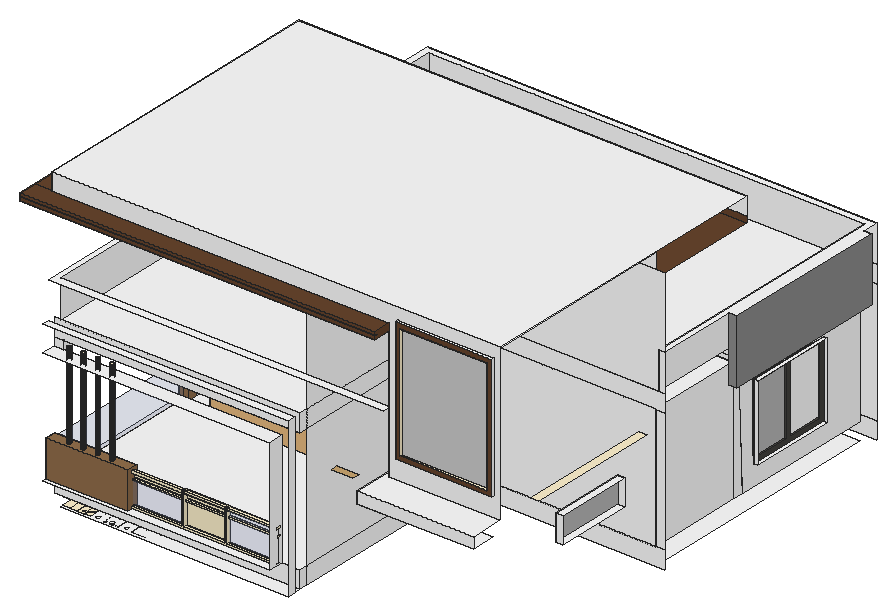
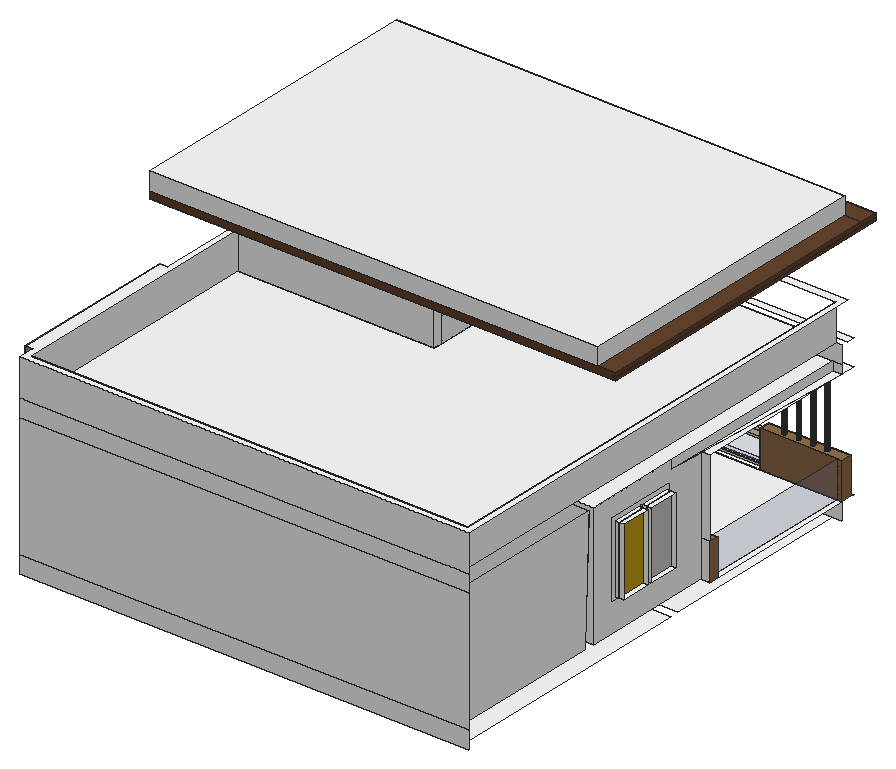
# SketchUp Ruby script. Lengths in inches.
U = 1.inch
M = Sketchup.active_model
def pt(a) = Geom::Point3d.new(a.map { |v| v * U })
def face(e, loops, mat)
  f = e.add_face(loops[0].map { |a| pt(a) })
  loops[1..].each { |l| e.add_face(l.map { |a| pt(a) }).erase! }
  f.material = f.back_material = mat if mat
  f
end
# faces: each face lists its corners as indices into pts; further lists are holes
def faces(e, pts, list, mat = nil) = list.each { |f| face(e, (f[0].is_a?(Array) ? f : [f]).map { |l| l.map { |i| pts[i] } }, mat) }
# xy, xz, yz: faces in a plane at the given z, y or x. An outline is a flat list of corners, or four numbers for a rectangle; further outlines are holes
def ring(l) = l.size == 4 ? [[l[0], l[1]], [l[2], l[1]], [l[2], l[3]], [l[0], l[3]]] : l.each_slice(2).to_a
def flat(e, list, mat, &to3) = list.each { |f| face(e, (f[0].is_a?(Array) ? f : [f]).map { |l| ring(l).map { |u, v| to3.(u, v) } }, mat) }
def xy(e, z, list, mat = nil) = flat(e, list, mat) { |x, y| [x, y, z] }
def xz(e, y, list, mat = nil) = flat(e, list, mat) { |x, z| [x, y, z] }
def yz(e, x, list, mat = nil) = flat(e, list, mat) { |y, z| [x, y, z] }
def lines(e, pts, list) = list.each { |a, b| e.add_line(pt(pts[a]), pt(pts[b])) }
# prism: a flat outline (further loops are holes) pulled along v
def prism(e, loops, v, mat = nil)
  f = face(e, loops, mat); d = Geom::Vector3d.new(v.map { |x| x * U })
  f.pushpull(f.normal.samedirection?(d) ? d.length : -d.length)
end
def box(e, o, s, mat = nil) = prism(e, [[o, [o[0] + s[0], o[1], o[2]], [o[0] + s[0], o[1] + s[1], o[2]], [o[0], o[1] + s[1], o[2]]]], [0, 0, s[2]], mat)
def at(x, y, z, deg = 0) = Geom::Transformation.translation(pt([x, y, z])) * Geom::Transformation.rotation(ORIGIN, Z_AXIS, deg.degrees)
def axes(o, x, y, z) = Geom::Transformation.new([*x, 0, *y, 0, *z, 0, *pt(o).to_a, 1])
def part(name) = M.definitions.add(name)
# library, detail: a bought-in or finely detailed component or shape, given as its bounding box
def library(name, o, s) = part(name).tap { |d| box(d.entities, o, s) }
def detail(e, o, s) = box(e.add_group.entities, o, s)
def put(e, d, t, mat = nil) = e.add_instance(d, t).tap { |i| i.material = mat if mat }
def group(e, t, mat = nil) = e.add_group.tap { |g| g.transformation = t; g.material = mat if mat }.entities
root = M.entities
M.materials.add("D01_Frost_White").color = [255, 242, 206]
M.materials.add("Glass_Mirror_01").color = [185, 185, 185]
M.materials.add("Glass_Sky Reflection_01").color = [126, 138, 183]
M.materials["Glass_Sky Reflection_01"].alpha = 0.25
M.materials.add("M00_Soft_Cloud").color = [255, 255, 255]
M.materials.add("M04_Stone_Frost").color = [142, 142, 142]
M.materials.add("Metal_06_1K").color = [238, 236, 231]
M.materials.add("Metal_Perforated_03_1K").color = [205, 205, 205]
M.materials.add("Metal_Perforated_08_1K").color = [201, 163, 22]
M.materials.add("Plywood_08_1K").color = [202, 166, 113]
M.materials.add("Wood_Floor_01_1K").color = [146, 111, 76]
M.materials.add("Wood_Planks_01_1K").color = [69, 67, 63]
M.materials.add("Wood_Veneer_15_1K1").color = [103, 69, 45]
c1 = library("michel-club1 (1)",[-34.67,-0.85,-0.13],[126.28,91.17,33.41])
xy(root,257.001,[[209.9258,109.0676,209.9294,119.6039],[209.933,109.0676,216.6168,119.6039],[216.6168,109.0676,223.3077,119.6039]],"D01_Frost_White")
xy(root,257.004,[[183.1639,109.0676,189.8512,119.6039],[189.8548,109.0676,196.5422,119.6039],[196.5529,109.0676,196.5547,119.6039]],"D01_Frost_White")
xy(root,257.0071,[[183.1621,109.0676,183.1657,119.6039],[196.5511,109.0676,203.242,119.6039],[203.242,109.0676,209.933,119.6039]],"D01_Frost_White")
xy(root,257.0132,[[169.7874,109.0676,176.4783,119.6039],[176.4783,109.0676,183.1692,119.6039]],"D01_Frost_White")
xy(root,257.0192,[[143.0236,109.0676,149.7146,119.6039],[149.7146,109.0676,156.4019,119.6039],[156.4055,109.0676,163.0929,119.6039],[163.0929,109.0676,169.7838,119.6039]],"D01_Frost_White")
xy(root,257.0192,[[[143.4397,105.8195,366,120],[190.0131,108.9163,189.5258,108.9804,189.0716,109.1685,188.6816,109.4678,188.3824,109.8578,188.1943,110.3119,188.1301,110.7993,188.1943,111.2867,188.3824,111.7408,188.6816,112.1308,189.0716,112.43,189.5258,112.6182,190.0131,112.6823,190.5005,112.6182,190.9547,112.43,191.3446,112.1308,191.6439,111.7408,191.832,111.2867,191.8962,110.7993,191.832,110.3119,191.6439,109.8578,191.3446,109.4678,190.9547,109.1685,190.5005,108.9804],[203.9218,108.9163,203.4345,108.9804,202.9803,109.1685,202.5903,109.4678,202.2911,109.8578,202.103,110.3119,202.0388,110.7993,202.103,111.2867,202.2911,111.7408,202.5903,112.1308,202.9803,112.43,203.4345,112.6182,203.9218,112.6823,204.4092,112.6182,204.8634,112.43,205.2534,112.1308,205.5526,111.7408,205.7407,111.2867,205.8049,110.7993,205.7407,110.3119,205.5526,109.8578,205.2534,109.4678,204.8634,109.1685,204.4092,108.9804],[162.1957,108.9163,161.7084,108.9804,161.2542,109.1685,160.8642,109.4678,160.565,109.8578,160.3769,110.3119,160.3127,110.7993,160.3769,111.2867,160.565,111.7408,160.8642,112.1308,161.2542,112.43,161.7084,112.6182,162.1957,112.6823,162.6831,112.6182,163.1373,112.43,163.5272,112.1308,163.8265,111.7408,164.0146,111.2867,164.0788,110.7993,164.0146,110.3119,163.8265,109.8578,163.5272,109.4678,163.1373,109.1685,162.6831,108.9804],[176.1044,108.9163,175.6171,108.9804,175.1629,109.1685,174.7729,109.4678,174.4737,109.8578,174.2856,110.3119,174.2214,110.7993,174.2856,111.2867,174.4737,111.7408,174.7729,112.1308,175.1629,112.43,175.6171,112.6182,176.1044,112.6823,176.5918,112.6182,177.046,112.43,177.4359,112.1308,177.7352,111.7408,177.9233,111.2867,177.9875,110.7993,177.9233,110.3119,177.7352,109.8578,177.4359,109.4678,177.046,109.1685,176.5918,108.9804]],[162.1957,108.9163,162.6831,108.9804,163.1373,109.1685,163.5272,109.4678,163.8265,109.8578,164.0146,110.3119,164.0788,110.7993,164.0146,111.2867,163.8265,111.7408,163.5272,112.1308,163.1373,112.43,162.6831,112.6182,162.1957,112.6823,161.7084,112.6182,161.2542,112.43,160.8642,112.1308,160.565,111.7408,160.3769,111.2867,160.3127,110.7993,160.3769,110.3119,160.565,109.8578,160.8642,109.4678,161.2542,109.1685,161.7084,108.9804],[176.1044,108.9163,176.5918,108.9804,177.046,109.1685,177.4359,109.4678,177.7352,109.8578,177.9233,110.3119,177.9875,110.7993,177.9233,111.2867,177.7352,111.7408,177.4359,112.1308,177.046,112.43,176.5918,112.6182,176.1044,112.6823,175.6171,112.6182,175.1629,112.43,174.7729,112.1308,174.4737,111.7408,174.2856,111.2867,174.2214,110.7993,174.2856,110.3119,174.4737,109.8578,174.7729,109.4678,175.1629,109.1685,175.6171,108.9804],[190.0131,108.9163,190.5005,108.9804,190.9547,109.1685,191.3446,109.4678,191.6439,109.8578,191.832,110.3119,191.8962,110.7993,191.832,111.2867,191.6439,111.7408,191.3446,112.1308,190.9547,112.43,190.5005,112.6182,190.0131,112.6823,189.5258,112.6182,189.0716,112.43,188.6816,112.1308,188.3824,111.7408,188.1943,111.2867,188.1301,110.7993,188.1943,110.3119,188.3824,109.8578,188.6816,109.4678,189.0716,109.1685,189.5258,108.9804],[203.9218,108.9163,204.4092,108.9804,204.8634,109.1685,205.2534,109.4678,205.5526,109.8578,205.7407,110.3119,205.8049,110.7993,205.7407,111.2867,205.5526,111.7408,205.2534,112.1308,204.8634,112.43,204.4092,112.6182,203.9218,112.6823,203.4345,112.6182,202.9803,112.43,202.5903,112.1308,202.2911,111.7408,202.103,111.2867,202.0388,110.7993,202.103,110.3119,202.2911,109.8578,202.5903,109.4678,202.9803,109.1685,203.4345,108.9804],
  [135,120,366,309],[135,318,555,567]],"M00_Soft_Cloud")
xy(root,274.0384,[[126,105.8195,348,105.8195,348,120,205.8751,120,205.8751,109.5496,126,109.5496],[126,109.5496,205.8751,120],[126,120,130.5,272.2237],[130.5,120,366,120,366,412.2579,135,412.2579,135,272.2237,130.5,272.2237],[126,272.2237,135,281.2237],
  [378.0564,318,555,412.2579]],"M00_Soft_Cloud")
xy(root,274.5723,[[205.8751,113.3173,348.7066,116.9059]],"D01_Frost_White")
xy(root,276.5176,[[205.8751,113.3173,255.4424,115.614],[257.6603,113.3173,297.4834,116.9059],[299.7013,113.3173,348.7066,115.1116],[299.7013,115.1116,348.7066,116.9059],[205.8751,115.614,255.4424,116.9059]],"D01_Frost_White")
xy(root,282.3496,[[366,337.9558,372.0282,371.4203],[372.0282,337.9558,378.0564,371.4203]],"M00_Soft_Cloud")
xy(root,298.6563,[[205.8751,114.3221,348.7066,116.9059]],"D01_Frost_White")
xy(root,298.8738,[[560.4663,430.9412,564,515.7903]],"M00_Soft_Cloud")
xy(root,300.1736,[[205.8751,114.3221,348.7066,116.9059]],"D01_Frost_White")
xy(root,302.8738,[[555,434.9412,557.7332,471.3657],[555,475.3657,557.7332,511.7903]],"M00_Soft_Cloud")
xy(root,302.8738,[[557.7332,434.9412,560.4663,471.3657],[557.7332,475.3657,560.4663,511.7903]],"Wood_Planks_01_1K")
xy(root,304.975,[[126,323.2546,130.5,353.0052],[130.5,323.2546,135,353.0052],[126,357.0052,130.5,386.7557],[130.5,357.0052,135,386.7557]],"M00_Soft_Cloud")
xy(root,305.9572,[[205.8751,113.3173,348.7066,116.9059]],"D01_Frost_White")
xy(root,307.9026,[[205.8751,113.3173,255.4424,116.9059],[255.4424,113.3173,257.6603,116.9059],[257.6603,113.3173,297.4834,116.9059],[297.4834,113.3173,299.7013,116.9059],[299.7013,113.3173,348.7066,116.9059]],"D01_Frost_White")
xy(root,310.0384,[[[126,109.5496,205.8751,120],[144.756,112.6463,144.2686,112.7104,143.8145,112.8986,143.4245,113.1978,143.1252,113.5878,142.9371,114.0419,142.873,114.5293,142.9371,115.0167,143.1252,115.4708,143.4245,115.8608,143.8145,116.1601,144.2686,116.3482,144.756,116.4123,145.2434,116.3482,145.6975,116.1601,146.0875,115.8608,146.3868,115.4708,146.5749,115.0167,146.639,114.5293,146.5749,114.0419,146.3868,113.5878,146.0875,113.1978,145.6975,112.8986,145.2434,112.7104],[158.6647,112.6463,158.1773,112.7104,157.7232,112.8986,157.3332,113.1978,157.034,113.5878,156.8458,114.0419,156.7817,114.5293,156.8458,115.0167,157.034,115.4708,157.3332,115.8608,157.7232,116.1601,158.1773,116.3482,158.6647,116.4123,159.1521,116.3482,159.6062,116.1601,159.9962,115.8608,160.2955,115.4708,160.4836,115.0167,160.5477,114.5293,160.4836,114.0419,160.2955,113.5878,159.9962,113.1978,159.6062,112.8986,159.1521,112.7104],[172.5734,112.6463,172.086,112.7104,171.6319,112.8986,171.2419,113.1978,170.9427,113.5878,170.7545,114.0419,170.6904,114.5293,170.7545,115.0167,170.9427,115.4708,171.2419,115.8608,171.6319,116.1601,172.086,116.3482,172.5734,116.4123,173.0608,116.3482,173.5149,116.1601,173.9049,115.8608,174.2042,115.4708,174.3923,115.0167,174.4564,114.5293,174.3923,114.0419,174.2042,113.5878,173.9049,113.1978,173.5149,112.8986,173.0608,112.7104],[186.4821,112.6463,185.9947,112.7104,185.5406,112.8986,185.1506,113.1978,184.8514,113.5878,184.6632,114.0419,184.5991,114.5293,184.6632,115.0167,184.8514,115.4708,185.1506,115.8608,185.5406,116.1601,185.9947,116.3482,186.4821,116.4123,186.9695,116.3482,187.4236,116.1601,187.8136,115.8608,188.1129,115.4708,188.301,115.0167,188.3651,114.5293,188.301,114.0419,188.1129,113.5878,187.8136,113.1978,187.4236,112.8986,186.9695,112.7104]],[126,272.2237,135,281.2237]],"Wood_Floor_01_1K")
xy(root,339.7221,[[564,184.6361,571,259.8187]],"M00_Soft_Cloud")
xy(root,364.3605,[[463.5996,116.0568,528.8247,122.5284],[463.5996,122.5284,528.8247,129]],"M00_Soft_Cloud")
xy(root,365.0444,[[564,184.6361,571,259.8187]],"M00_Soft_Cloud")
xy(root,368.9179,[[555,434.9412,557.7332,471.3657],[555,475.3657,557.7332,511.7903]],"M00_Soft_Cloud")
xy(root,368.9179,[[557.7332,434.9412,560.4663,471.3657],[557.7332,475.3657,560.4663,511.7903]],"Wood_Planks_01_1K")
xy(root,371.0202,[[366,337.9558,372.0282,371.4203],[372.0282,337.9558,378.0564,371.4203]],"M00_Soft_Cloud")
xy(root,371.1879,[[126,323.2546,130.5,353.0052],[130.5,323.2546,135,353.0052],[126,357.0052,130.5,386.7557],[130.5,357.0052,135,386.7557]],"M00_Soft_Cloud")
xy(root,372.3605,[[455.5996,116.0568,536.8247,128.0311]],"M00_Soft_Cloud")
xy(root,372.9179,[[560.4663,430.9412,564,515.7903]],"M00_Soft_Cloud")
xy(root,377.4389,[[450.4407,84.0124,450.4407,128.0311,546,128.0311,546,108.0124,564,108.0124,564,84.0124]],"M00_Soft_Cloud")
xy(root,377.6765,[[402.037,112.9098,423.1418,120]],"Plywood_08_1K")
xy(root,384.3022,[[564,396.1656,571.6233,560.6941]],"M04_Stone_Frost")
xy(root,385.4776,[[126,105.8195,348,120]],"M00_Soft_Cloud")
xy(root,388.7049,[[450.4407,84.0124,564,84.0124,564,116.3941,455.5996,116.3941,455.5996,128.0311,450.4407,128.0311]],"M00_Soft_Cloud")
xy(root,390.9895,[[564,154.6118,571,286.5421]],"D01_Frost_White")
xy(root,394.0384,[[144.756,112.6463,145.2434,112.7104,145.6975,112.8986,146.0875,113.1978,146.3868,113.5878,146.5749,114.0419,146.639,114.5293,146.5749,115.0167,146.3868,115.4708,146.0875,115.8608,145.6975,116.1601,145.2434,116.3482,144.756,116.4123,144.2686,116.3482,143.8145,116.1601,143.4245,115.8608,143.1252,115.4708,142.9371,115.0167,142.873,114.5293,142.9371,114.0419,143.1252,113.5878,143.4245,113.1978,143.8145,112.8986,144.2686,112.7104],[158.6647,112.6463,159.1521,112.7104,159.6062,112.8986,159.9962,113.1978,160.2955,113.5878,160.4836,114.0419,160.5477,114.5293,160.4836,115.0167,160.2955,115.4708,159.9962,115.8608,159.6062,116.1601,159.1521,116.3482,158.6647,116.4123,158.1773,116.3482,157.7232,116.1601,157.3332,115.8608,157.034,115.4708,156.8458,115.0167,156.7817,114.5293,156.8458,114.0419,157.034,113.5878,157.3332,113.1978,157.7232,112.8986,158.1773,112.7104],[172.5734,112.6463,173.0608,112.7104,173.5149,112.8986,173.9049,113.1978,174.2042,113.5878,174.3923,114.0419,174.4564,114.5293,174.3923,115.0167,174.2042,115.4708,173.9049,115.8608,173.5149,116.1601,173.0608,116.3482,172.5734,116.4123,172.086,116.3482,171.6319,116.1601,171.2419,115.8608,170.9427,115.4708,170.7545,115.0167,170.6904,114.5293,170.7545,114.0419,170.9427,113.5878,171.2419,113.1978,171.6319,112.8986,172.086,112.7104],[186.4821,112.6463,186.9695,112.7104,187.4236,112.8986,187.8136,113.1978,188.1129,113.5878,188.301,114.0419,188.3651,114.5293,188.301,115.0167,188.1129,115.4708,187.8136,115.8608,187.4236,116.1601,186.9695,116.3482,186.4821,116.4123,185.9947,116.3482,185.5406,116.1601,185.1506,115.8608,184.8514,115.4708,184.6632,115.0167,184.5991,114.5293,184.6632,114.0419,184.8514,113.5878,185.1506,113.1978,185.5406,112.8986,185.9947,112.7104]],"D01_Frost_White")
xy(root,394.0384,[[135,120,366,412.2579],[378.0564,318,555,412.2579]],"M00_Soft_Cloud")
xy(root,408.2202,[[464.2846,113.3941,558.2295,116.3941]],"M00_Soft_Cloud")
xy(root,411.0577,[[126,105.8195,366,112.9098],[132,120,366,120,366,318,558,318,558,570,132,570]],"M00_Soft_Cloud")
xy(root,412.4676,[[468.532,113.3941,553.9822,116.3941]],"D01_Frost_White")
xy(root,447.0577,[[126,112.9098,453.2434,112.9098,453.2434,120,132,120,132,570,558,570,558,318,564,318,564,396.1656,571.6233,396.1656,571.6233,560.6941,564,560.6941,564,576,126,576]],"M00_Soft_Cloud")
xy(root,516.2435,[[[109.1309,99.1487,109.1309,417.7283,564,417.7283,564,318,366,318,366,128.0311,455.5996,128.0311,455.5996,99.1487],[152.3218,168.8733,170.5166,192.8121]]],"Wood_Veneer_15_1K1")
xy(root,519.1637,[[109.1309,99.1487,455.5996,102.1487],[109.1309,102.1487,112.1309,417.7283]],"D01_Frost_White")
xy(root,520.1637,[[109.1309,102.1487,112.1309,417.7283]],"D01_Frost_White")
xy(root,520.1637,[[109.1309,99.1487,455.5996,102.1487]],"Wood_Veneer_15_1K1")
xy(root,523.0839,[[109.1309,99.1487,455.5996,116.3941],[109.1309,116.3941,126,417.7283]],"Wood_Veneer_15_1K1")
xy(root,524.3175,[[468.532,113.3941,553.9822,116.3941]],"Wood_Veneer_15_1K1")
xy(root,528.5649,[[464.2846,113.3941,558.2295,116.3941]],"M00_Soft_Cloud")
xy(root,531.0577,[[375,129,555,309],[366,309,375,318],[375,309,555,318]],"M00_Soft_Cloud")
xy(root,540.0577,[[126,116.3941,564,417.7283]],"M00_Soft_Cloud")
xz(root,84.0124,[[450.4407,377.4389,564,388.7049]],"M00_Soft_Cloud")
xz(root,99.1487,[[109.1309,516.2435,455.5996,519.1637],[109.1309,520.1637,455.5996,523.0839]],"Wood_Veneer_15_1K1")
xz(root,102.1487,[[112.1309,519.1637,455.5996,520.1637]],"D01_Frost_White")
xz(root,109.0676,[[196.5618,256.9888,196.5547,257.001,196.5547,257.001],[209.933,256.9889,209.933,257.001,209.9294,257.001,209.9276,256.998],[209.9276,256.998,209.9294,257.001,209.9258,257.001],[196.5547,257.001,196.5547,257.001,196.5529,257.004,196.5529,257.004],[196.5547,257.001,196.5547,257.004,196.5529,257.004],
  [209.9294,257.001,209.933,257.001,209.933,257.0071],[183.1639,257.004,183.1657,257.0071,183.1621,257.0071],[183.1639,257.004,189.8512,257.004,189.853,257.0071,183.1657,257.0071],[189.8512,257.004,189.8548,257.004,189.853,257.0071],[189.8548,257.004,196.5422,257.004,196.544,257.0071,189.853,257.0071],
  [196.5493,257.004,196.5529,257.004,196.5511,257.0071],[196.5529,257.004,196.5529,257.004,196.5511,257.0071],[156.4037,257.0162,156.4055,257.0192,156.4019,257.0192]],"D01_Frost_White")
xz(root,109.5496,[[126,274.0384,205.8751,310.0384]],"Wood_Floor_01_1K")
xz(root,113.3173,[[205.8751,274.5723,348.7066,274.5723,348.7066,276.5176,299.7013,276.5176,299.7013,305.9572,297.4834,305.9572,297.4834,276.5176,257.6603,276.5176,257.6603,305.9572,255.4424,305.9572,255.4424,276.5176,205.8751,276.5176],[205.8751,305.9572,255.4424,307.9026],[255.4424,305.9572,257.6603,307.9026],[257.6603,305.9572,297.4834,307.9026],[297.4834,305.9572,299.7013,307.9026],
  [299.7013,305.9572,348.7066,307.9026]],"D01_Frost_White")
xz(root,113.3941,[[[464.2846,408.2202,558.2295,528.5649],[468.532,412.4676,553.9822,524.3175]]],"Wood_Veneer_15_1K1")
xz(root,114.3221,[[205.8751,298.6563,348.7066,300.1736]],"D01_Frost_White")
xz(root,115.1116,[[299.7013,276.5176,348.7066,305.9572]],"Glass_Sky Reflection_01")
xz(root,115.614,[[205.8751,276.5176,255.4424,298.6563]],"Glass_Sky Reflection_01")
xz(root,116.3941,[[[455.5996,388.7049,564,388.7049,564,540.0577,126,540.0577,126,523.0839,455.5996,523.0839],[464.2846,408.2202,558.2295,528.5649]]],"M00_Soft_Cloud")
xz(root,116.3941,[[468.532,412.4676,553.9822,524.3175]],"Metal_Perforated_03_1K")
xz(root,116.9059,[[205.8751,274.5723,205.8751,276.5176,255.4424,276.5176,255.4424,298.6563,257.6603,298.6563,257.6603,276.5176,297.4834,276.5176,297.4834,298.6563,299.7013,298.6563,299.7013,276.5176,348.7066,276.5176,348.7066,274.5723],[257.6603,276.5176,297.4834,298.6563],[205.8751,298.6563,255.4424,300.1736],[255.4424,298.6563,257.6603,300.1736],[257.6603,298.6563,297.4834,300.1736],
  [297.4834,298.6563,299.7013,300.1736],[299.7013,298.6563,348.7066,300.1736],[205.8751,300.1736,255.4424,305.9572],[255.4424,300.1736,257.6603,305.9572],[257.6603,300.1736,297.4834,305.9572],
  [297.4834,300.1736,299.7013,305.9572],[205.8751,305.9572,255.4424,307.9026],[255.4424,305.9572,257.6603,307.9026],[257.6603,305.9572,297.4834,307.9026],[297.4834,305.9572,299.7013,307.9026],
  [299.7013,305.9572,348.7066,307.9026]],"D01_Frost_White")
xz(root,120,[[126,257.0192,366,274.0384],[126,385.4844,135,394.0384],[126,394.0384,366,411.0577]],"M00_Soft_Cloud")
xz(root,120,[[126,274.0384,130.5,310.0384],[130.5,274.0384,205.8751,310.0384]],"Wood_Floor_01_1K")
xz(root,184.6361,[[564,339.7221,571,365.0444]],"M00_Soft_Cloud")
xz(root,259.8187,[[564,339.7221,571,365.0444]],"M00_Soft_Cloud")
xz(root,272.2237,[[126,274.0384,130.5,310.0384],[130.5,274.0384,135,310.0384]],"Wood_Floor_01_1K")
xz(root,281.2237,[[126,274.0384,135,310.0384],[126,310.0384,135,310.0384,135,385.4844,133.6773,385.4841,126,385.4844]],"M00_Soft_Cloud")
xz(root,309,[[366,411.0577,375,531.0577]],"M00_Soft_Cloud")
xz(root,318,[[366,257.0192,564,274.0384],[366,274.0384,378.0564,394.0384],[378.0564,274.0384,555,394.0384],[555,274.0384,564,394.0384],[366,394.0384,564,411.0577],
  [366,411.0577,366,516.2435,564,516.2435,564,447.0577,558,447.0577,558,411.0577],[558,411.0577,564,447.0577],[366,516.2435,375,531.0577],[375,516.2435,555,531.0577]],"M00_Soft_Cloud")
xz(root,323.2546,[[126,304.975,130.5,371.1879],[130.5,304.975,135,371.1879]],"M00_Soft_Cloud")
xz(root,337.9558,[[366,282.3496,372.0282,371.0202],[372.0282,282.3496,378.0564,371.0202]],"M00_Soft_Cloud")
xz(root,353.0052,[[126,304.975,130.5,371.1879],[130.5,304.975,135,371.1879]],"M00_Soft_Cloud")
xz(root,357.0052,[[126,304.975,130.5,371.1879],[130.5,304.975,135,371.1879]],"M00_Soft_Cloud")
xz(root,371.4203,[[366,282.3496,372.0282,371.0202],[372.0282,282.3496,378.0564,371.0202]],"M00_Soft_Cloud")
xz(root,386.7557,[[126,304.975,130.5,371.1879],[130.5,304.975,135,371.1879]],"M00_Soft_Cloud")
xz(root,396.1656,[[564,384.3022,571.6233,447.0577]],"M04_Stone_Frost")
xz(root,412.2579,[[135,274.0384,366,394.0384],[378.0564,274.0384,555,394.0384]],"M00_Soft_Cloud")
xz(root,417.7283,[[126,523.0839,564,540.0577]],"M00_Soft_Cloud")
xz(root,417.7283,[[109.1309,516.2435,109.1309,519.1637,112.1309,519.1637,112.1309,520.1637,109.1309,520.1637,109.1309,523.0839,564,523.0839,564,516.2435]],"Wood_Veneer_15_1K1")
xz(root,430.9412,[[560.4663,298.8738,564,372.9179]],"M00_Soft_Cloud")
xz(root,434.9412,[[555,302.8738,557.7332,368.9179]],"M00_Soft_Cloud")
xz(root,434.9412,[[557.7332,302.8738,560.4663,368.9179]],"Wood_Planks_01_1K")
xz(root,471.3657,[[555,302.8738,557.7332,368.9179]],"M00_Soft_Cloud")
xz(root,471.3657,[[557.7332,302.8738,560.4663,368.9179]],"Wood_Planks_01_1K")
xz(root,475.3657,[[555,302.8738,557.7332,368.9179]],"M00_Soft_Cloud")
xz(root,475.3657,[[557.7332,302.8738,560.4663,368.9179]],"Wood_Planks_01_1K")
xz(root,511.7903,[[555,302.8738,557.7332,368.9179]],"M00_Soft_Cloud")
xz(root,511.7903,[[557.7332,302.8738,560.4663,368.9179]],"Wood_Planks_01_1K")
xz(root,515.7903,[[560.4663,298.8738,564,372.9179]],"M00_Soft_Cloud")
xz(root,560.6941,[[564,384.3022,571.6233,447.0577]],"M04_Stone_Frost")
xz(root,567,[[135,274.0384,555,394.0384]],"M00_Soft_Cloud")
xz(root,570,[[132,411.0577,558,447.0577]],"M00_Soft_Cloud")
xz(root,576,[[126,257.0192,564,274.0384],[126,274.0384,564,394.0384],[126,394.0384,564,411.0577],[126,411.0577,564,447.0577]],"M00_Soft_Cloud")
yz(root,109.1309,[[99.1487,516.2435,417.7283,519.1637],[99.1487,520.1637,417.7283,523.0839]],"Wood_Veneer_15_1K1")
yz(root,112.1309,[[102.1487,519.1637,417.7283,520.1637]],"D01_Frost_White")
yz(root,126,[[116.3941,523.0839,417.7283,540.0577]],"M00_Soft_Cloud")
yz(root,126,[[109.5496,274.0384,120,310.0384],[272.2237,274.0384,281.2237,310.0384]],"Wood_Floor_01_1K")
yz(root,130.5,[[120,274.0384,272.2237,310.0384]],"Glass_Sky Reflection_01")
yz(root,130.5,[[323.2546,304.975,353.0052,371.1879]],"Metal_Perforated_03_1K")
yz(root,130.5,[[357.0052,304.975,386.7557,371.1879]],"Metal_Perforated_08_1K")
yz(root,132,[[120,411.0577,570,447.0577]],"M00_Soft_Cloud")
yz(root,135,[[[281.2237,274.0384,412.2579,274.0384,412.2579,394.0384,318,394.0384,318,385.4844,281.2237,385.4844],[319.2546,300.975,390.7557,375.1879]],[422.648,274.0384,567,274.0384,567,394.0384,418.4476,394.0384],[[319.2546,300.975,390.7557,375.1879],[323.2546,304.975,386.7557,371.1879]],[353.0052,304.975,357.0052,371.1879],[120,385.4844,318,394.0384]],"M00_Soft_Cloud")
yz(root,135,[[272.2237,274.0384,281.2237,310.0384]],"Wood_Floor_01_1K")
yz(root,196.5547,[[109.0676,257.001,119.6039,257.004]],"D01_Frost_White")
yz(root,205.8751,[[[109.5496,274.0384,120,310.0384],[113.3173,305.9572,116.9059,307.9026]]],"Wood_Floor_01_1K")
yz(root,209.933,[[109.0676,256.9889,119.6039,257.001]],"D01_Frost_White")
yz(root,255.4424,[[113.3173,276.5176,116.9059,307.9026]],"D01_Frost_White")
yz(root,257.6603,[[113.3173,276.5176,116.9059,307.9026]],"D01_Frost_White")
yz(root,297.4834,[[113.3173,276.5176,116.9059,307.9026]],"D01_Frost_White")
yz(root,299.7013,[[113.3173,276.5176,116.9059,307.9026]],"D01_Frost_White")
yz(root,348,[[105.8195,274.0384,120,385.4776]],"M00_Soft_Cloud")
yz(root,348.7066,[[114.3221,298.6563,115.1116,300.1736],[115.1116,298.6563,116.9059,300.1736],[113.3173,305.9572,116.9059,307.9026]],"D01_Frost_White")
yz(root,366,[[105.8195,257.0192,112.9098,411.0577],[120,257.0192,128.0311,274.0384],[128.0311,257.0192,309,274.0384],[309,257.0192,318,274.0384],[128.0311,274.0384,309,394.0384],
  [309,274.0384,318,394.0384],[[318,274.0384,412.2579,394.0384],[334.1505,282.3496,373.7105,374.8254]],[120,394.0384,128.0311,411.0577],[128.0311,394.0384,309,411.0577],[309,394.0384,318,411.0577],
  [128.0311,411.0577,309,516.2435],[309,411.0577,318,516.2435],[309,516.2435,318,531.0577]],"M00_Soft_Cloud")
yz(root,366,[[334.1505,282.3496,334.1505,374.8254,373.7105,374.8254,373.7105,282.3496,371.4203,282.3496,371.4203,371.0202,337.9558,371.0202,337.9558,282.3496]],"Wood_Planks_01_1K")
yz(root,372.0282,[[337.9558,282.3496,371.4203,371.0202]],"Wood_Veneer_15_1K1")
yz(root,378.0564,[[[318,274.0384,412.2579,394.0384],[337.9558,282.3496,371.4203,371.0202]]],"M00_Soft_Cloud")
yz(root,450.4407,[[84.0124,377.4389,128.0311,388.7049]],"M00_Soft_Cloud")
yz(root,455.5996,[[116.3941,388.7049,128.0311,516.2435]],"M00_Soft_Cloud")
yz(root,455.5996,[[99.1487,516.2435,116.3941,516.2435,116.3941,523.0839,99.1487,523.0839,99.1487,520.1637,102.1487,520.1637,102.1487,519.1637,99.1487,519.1637]],"Wood_Veneer_15_1K1")
yz(root,464.2846,[[113.3941,408.2202,116.3941,528.5649]],"M00_Soft_Cloud")
yz(root,468.532,[[113.3941,412.4676,116.3941,524.3175]],"D01_Frost_White")
yz(root,553.9822,[[113.3941,412.4676,116.3941,524.3175]],"D01_Frost_White")
yz(root,555,[[318,274.0384,412.2579,394.0384],[412.2579,274.0384,422.648,274.0384,418.4476,394.0384,412.2579,394.0384],[[422.648,274.0384,418.4476,394.0384,567,394.0384,567,274.0384],[475.3657,302.8738,511.7903,368.9179],[434.9412,302.8738,471.3657,368.9179]]],"M00_Soft_Cloud")
yz(root,557.7332,[[434.9412,302.8738,471.3657,368.9179]],"Glass_Mirror_01")
yz(root,557.7332,[[475.3657,302.8738,511.7903,368.9179]],"M00_Soft_Cloud")
yz(root,558,[[318,411.0577,570,447.0577]],"M00_Soft_Cloud")
yz(root,558.2295,[[113.3941,408.2202,116.3941,528.5649]],"M00_Soft_Cloud")
yz(root,560.4663,[[[430.9412,298.8738,515.7903,372.9179],[475.3657,302.8738,511.7903,368.9179],[434.9412,302.8738,471.3657,368.9179]]],"Wood_Planks_01_1K")
yz(root,564,[[184.6361,339.7221,259.8187,365.0444]],"Glass_Mirror_01")
yz(root,571.6233,[[396.1656,384.3022,560.6941,447.0577]],"M04_Stone_Frost")
p = [[156.4037,109.0676,257.0162],[156.4019,109.0676,257.0192],[156.4019,119.6039,257.0192],[156.4037,119.6039,257.0162],[156.4055,109.0676,257.0192],[156.4055,119.6039,257.0192],
  [183.1639,109.0676,257.004],[183.1621,109.0676,257.0071],[183.1621,119.6039,257.0071],[183.1639,119.6039,257.004],[183.1657,109.0676,257.0071],[183.1692,109.0676,257.0132],
  [183.1692,119.6039,257.0132],[183.1657,119.6039,257.0071],[196.5511,109.0676,257.0071],[196.5529,109.0676,257.004],[196.5529,119.6039,257.004],[196.5511,119.6039,257.0071],
  [209.9276,109.0676,256.998],[209.9258,109.0676,257.001],[209.9258,119.6039,257.001],[209.9276,119.6039,256.998],[209.9294,109.0676,257.001],[209.933,109.0676,257.0071],
  [209.933,119.6039,257.0071],[209.9294,119.6039,257.001],[135,422.648,274.0384],[135,418.4476,394.0384],[555,418.4476,394.0384],[555,422.648,274.0384],
  [144.2686,112.7104,310.0384],[144.756,112.6463,310.0384],[144.756,112.6463,394.0384],[144.2686,112.7104,394.0384],[145.2434,112.7104,310.0384],[145.2434,112.7104,394.0384],
  [158.1773,112.7104,310.0384],[158.6647,112.6463,310.0384],[158.6647,112.6463,394.0384],[158.1773,112.7104,394.0384],[159.1521,112.7104,310.0384],[159.1521,112.7104,394.0384],
  [172.086,112.7104,310.0384],[172.5734,112.6463,310.0384],[172.5734,112.6463,394.0384],[172.086,112.7104,394.0384],[173.0608,112.7104,310.0384],[173.0608,112.7104,394.0384],
  [185.9947,112.7104,310.0384],[186.4821,112.6463,310.0384],[186.4821,112.6463,394.0384],[185.9947,112.7104,394.0384],[186.9695,112.7104,310.0384],[186.9695,112.7104,394.0384],
  [143.8145,112.8986,310.0384],[143.8145,112.8986,394.0384],[145.6975,112.8986,310.0384],[145.6975,112.8986,394.0384],[157.7232,112.8986,310.0384],[157.7232,112.8986,394.0384],
  [159.6062,112.8986,310.0384],[159.6062,112.8986,394.0384],[171.6319,112.8986,310.0384],[171.6319,112.8986,394.0384],[173.5149,112.8986,310.0384],[173.5149,112.8986,394.0384],
  [185.5406,112.8986,310.0384],[185.5406,112.8986,394.0384],[187.4236,112.8986,310.0384],[187.4236,112.8986,394.0384],[143.4245,113.1978,310.0384],[143.4245,113.1978,394.0384],
  [146.0875,113.1978,310.0384],[146.0875,113.1978,394.0384],[157.3332,113.1978,310.0384],[157.3332,113.1978,394.0384],[159.9962,113.1978,310.0384],[159.9962,113.1978,394.0384],
  [171.2419,113.1978,310.0384],[171.2419,113.1978,394.0384],[173.9049,113.1978,310.0384],[173.9049,113.1978,394.0384],[185.1506,113.1978,310.0384],[185.1506,113.1978,394.0384],
  [187.8136,113.1978,310.0384],[187.8136,113.1978,394.0384],[143.1252,113.5878,310.0384],[143.1252,113.5878,394.0384],[146.3868,113.5878,310.0384],[146.3868,113.5878,394.0384],
  [157.034,113.5878,310.0384],[157.034,113.5878,394.0384],[160.2955,113.5878,310.0384],[160.2955,113.5878,394.0384],[170.9427,113.5878,310.0384],[170.9427,113.5878,394.0384],
  [174.2042,113.5878,310.0384],[174.2042,113.5878,394.0384],[184.8514,113.5878,310.0384],[184.8514,113.5878,394.0384],[188.1129,113.5878,310.0384],[188.1129,113.5878,394.0384],
  [142.9371,114.0419,310.0384],[142.9371,114.0419,394.0384],[146.5749,114.0419,310.0384],[146.5749,114.0419,394.0384],[156.8458,114.0419,310.0384],[156.8458,114.0419,394.0384],
  [160.4836,114.0419,310.0384],[160.4836,114.0419,394.0384],[170.7545,114.0419,310.0384],[170.7545,114.0419,394.0384],[174.3923,114.0419,310.0384],[174.3923,114.0419,394.0384],
  [184.6632,114.0419,310.0384],[184.6632,114.0419,394.0384],[188.301,114.0419,310.0384],[188.301,114.0419,394.0384],[142.873,114.5293,310.0384],[142.873,114.5293,394.0384],
  [146.639,114.5293,310.0384],[146.639,114.5293,394.0384],[156.7817,114.5293,310.0384],[156.7817,114.5293,394.0384],[160.5477,114.5293,310.0384],[160.5477,114.5293,394.0384],
  [170.6904,114.5293,310.0384],[170.6904,114.5293,394.0384],[174.4564,114.5293,310.0384],[174.4564,114.5293,394.0384],[184.5991,114.5293,310.0384],[184.5991,114.5293,394.0384],
  [188.3651,114.5293,310.0384],[188.3651,114.5293,394.0384],[142.9371,115.0167,310.0384],[142.9371,115.0167,394.0384],[146.5749,115.0167,310.0384],[146.5749,115.0167,394.0384],
  [156.8458,115.0167,310.0384],[156.8458,115.0167,394.0384],[160.4836,115.0167,310.0384],[160.4836,115.0167,394.0384],[170.7545,115.0167,310.0384],[170.7545,115.0167,394.0384],
  [174.3923,115.0167,310.0384],[174.3923,115.0167,394.0384],[184.6632,115.0167,310.0384],[184.6632,115.0167,394.0384],[188.301,115.0167,310.0384],[188.301,115.0167,394.0384],
  [143.1252,115.4708,310.0384],[143.1252,115.4708,394.0384],[146.3868,115.4708,310.0384],[146.3868,115.4708,394.0384],[157.034,115.4708,310.0384],[157.034,115.4708,394.0384],
  [160.2955,115.4708,310.0384],[160.2955,115.4708,394.0384],[170.9427,115.4708,310.0384],[170.9427,115.4708,394.0384],[174.2042,115.4708,310.0384],[174.2042,115.4708,394.0384],
  [184.8514,115.4708,310.0384],[184.8514,115.4708,394.0384],[188.1129,115.4708,310.0384],[188.1129,115.4708,394.0384],[143.4245,115.8608,310.0384],[143.4245,115.8608,394.0384],
  [146.0875,115.8608,310.0384],[146.0875,115.8608,394.0384],[157.3332,115.8608,310.0384],[157.3332,115.8608,394.0384],[159.9962,115.8608,310.0384],[159.9962,115.8608,394.0384],
  [171.2419,115.8608,310.0384],[171.2419,115.8608,394.0384],[173.9049,115.8608,310.0384],[173.9049,115.8608,394.0384],[185.1506,115.8608,310.0384],[185.1506,115.8608,394.0384],
  [187.8136,115.8608,310.0384],[187.8136,115.8608,394.0384],[143.8145,116.1601,310.0384],[143.8145,116.1601,394.0384],[145.6975,116.1601,310.0384],[145.6975,116.1601,394.0384],
  [157.7232,116.1601,310.0384],[157.7232,116.1601,394.0384],[159.6062,116.1601,310.0384],[159.6062,116.1601,394.0384],[171.6319,116.1601,310.0384],[171.6319,116.1601,394.0384],
  [173.5149,116.1601,310.0384],[173.5149,116.1601,394.0384],[185.5406,116.1601,310.0384],[185.5406,116.1601,394.0384],[187.4236,116.1601,310.0384],[187.4236,116.1601,394.0384],
  [144.2686,116.3482,310.0384],[144.2686,116.3482,394.0384],[145.2434,116.3482,310.0384],[145.2434,116.3482,394.0384],[158.1773,116.3482,310.0384],[158.1773,116.3482,394.0384],
  [159.1521,116.3482,310.0384],[159.1521,116.3482,394.0384],[172.086,116.3482,310.0384],[172.086,116.3482,394.0384],[173.0608,116.3482,310.0384],[173.0608,116.3482,394.0384],
  [185.9947,116.3482,310.0384],[185.9947,116.3482,394.0384],[186.9695,116.3482,310.0384],[186.9695,116.3482,394.0384],[144.756,116.4123,310.0384],[144.756,116.4123,394.0384],
  [158.6647,116.4123,310.0384],[158.6647,116.4123,394.0384],[172.5734,116.4123,310.0384],[172.5734,116.4123,394.0384],[186.4821,116.4123,310.0384],[186.4821,116.4123,394.0384],
  [133.6773,281.2237,385.4841],[135,281.2237,385.4844],[135,120,385.4844],[126,120,385.4844],[126,281.2237,385.4844],[126,120,385.4776],
  [134.1429,291,385.4841],[135,309,385.4844],[223.3148,109.0676,257.0071]]
faces(root,p,[[0,1,2,3],[4,0,3,5],[6,7,8,9],[10,11,12,13],[14,15,16,17],[18,19,20,21],[22,23,24,25]],"D01_Frost_White")
faces(root,p,[[26,27,28,29],[222,223,224,225,226]],"M00_Soft_Cloud")
faces(root,p,[[30,31,32,33],[31,34,35,32],[36,37,38,39],[37,40,41,38],[42,43,44,45],[43,46,47,44],[48,49,50,51],[49,52,53,50],
  [54,30,33,55],[34,56,57,35],[58,36,39,59],[40,60,61,41],[62,42,45,63],[46,64,65,47],[66,48,51,67],[52,68,69,53],
  [70,54,55,71],[56,72,73,57],[74,58,59,75],[60,76,77,61],[78,62,63,79],[64,80,81,65],[82,66,67,83],[68,84,85,69],
  [86,70,71,87],[72,88,89,73],[90,74,75,91],[76,92,93,77],[94,78,79,95],[80,96,97,81],[98,82,83,99],[84,100,101,85],
  [102,86,87,103],[88,104,105,89],[106,90,91,107],[92,108,109,93],[110,94,95,111],[96,112,113,97],[114,98,99,115],[100,116,117,101],
  [118,102,103,119],[104,120,121,105],[122,106,107,123],[108,124,125,109],[126,110,111,127],[112,128,129,113],[130,114,115,131],[116,132,133,117],
  [134,118,119,135],[120,136,137,121],[138,122,123,139],[124,140,141,125],[142,126,127,143],[128,144,145,129],[146,130,131,147],[132,148,149,133],
  [150,134,135,151],[136,152,153,137],[154,138,139,155],[140,156,157,141],[158,142,143,159],[144,160,161,145],[162,146,147,163],[148,164,165,149],
  [166,150,151,167],[152,168,169,153],[170,154,155,171],[156,172,173,157],[174,158,159,175],[160,176,177,161],[178,162,163,179],[164,180,181,165],
  [182,166,167,183],[168,184,185,169],[186,170,171,187],[172,188,189,173],[190,174,175,191],[176,192,193,177],[194,178,179,195],[180,196,197,181],
  [198,182,183,199],[184,200,201,185],[202,186,187,203],[188,204,205,189],[206,190,191,207],[192,208,209,193],[210,194,195,211],[196,212,213,197],
  [214,198,199,215],[200,214,215,201],[216,202,203,217],[204,216,217,205],[218,206,207,219],[208,218,219,209],[220,210,211,221],[212,220,221,213]],"Metal_06_1K")
lines(root,p,[[227,222],[228,229],[222,228],[230,23]])
put(root,c1,axes([202.2,264.125,274.1],[1.14,0,0],[0,1,0],[0,0,1.48]))
